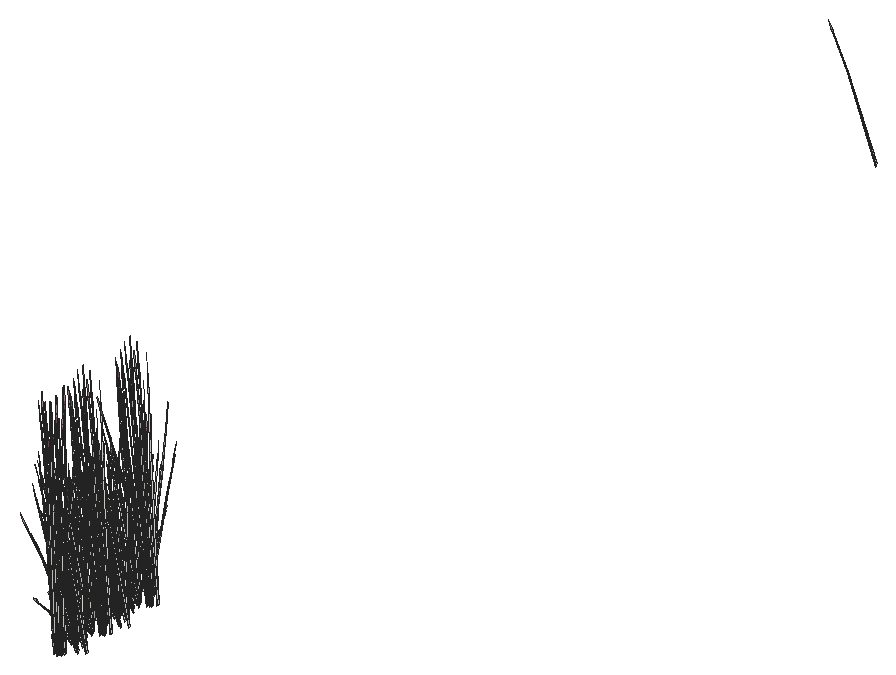
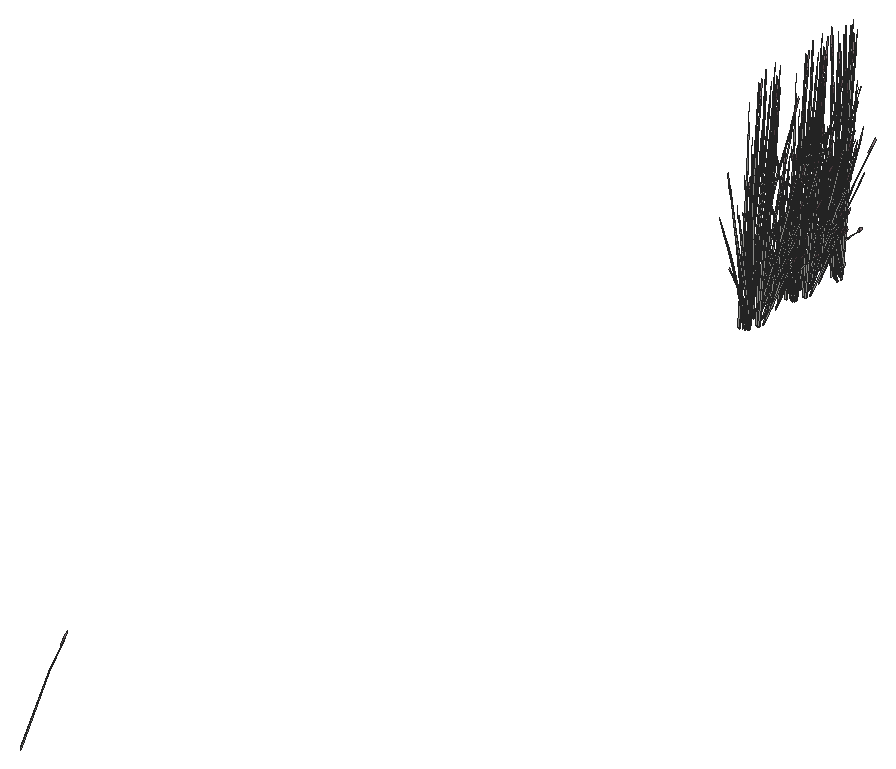
# SketchUp Ruby script. Lengths in inches.
U = 1.inch
M = Sketchup.active_model
def pt(a) = Geom::Point3d.new(a.map { |v| v * U })
def face(e, loops, mat)
  f = e.add_face(loops[0].map { |a| pt(a) })
  loops[1..].each { |l| e.add_face(l.map { |a| pt(a) }).erase! }
  f.material = f.back_material = mat if mat
  f
end
# faces: each face lists its corners as indices into pts; further lists are holes
def faces(e, pts, list, mat = nil) = list.each { |f| face(e, (f[0].is_a?(Array) ? f : [f]).map { |l| l.map { |i| pts[i] } }, mat) }
# xy, xz, yz: faces in a plane at the given z, y or x. An outline is a flat list of corners, or four numbers for a rectangle; further outlines are holes
def ring(l) = l.size == 4 ? [[l[0], l[1]], [l[2], l[1]], [l[2], l[3]], [l[0], l[3]]] : l.each_slice(2).to_a
def flat(e, list, mat, &to3) = list.each { |f| face(e, (f[0].is_a?(Array) ? f : [f]).map { |l| ring(l).map { |u, v| to3.(u, v) } }, mat) }
def xy(e, z, list, mat = nil) = flat(e, list, mat) { |x, y| [x, y, z] }
def xz(e, y, list, mat = nil) = flat(e, list, mat) { |x, z| [x, y, z] }
def yz(e, x, list, mat = nil) = flat(e, list, mat) { |y, z| [x, y, z] }
def lines(e, pts, list) = list.each { |a, b| e.add_line(pt(pts[a]), pt(pts[b])) }
# prism: a flat outline (further loops are holes) pulled along v
def prism(e, loops, v, mat = nil)
  f = face(e, loops, mat); d = Geom::Vector3d.new(v.map { |x| x * U })
  f.pushpull(f.normal.samedirection?(d) ? d.length : -d.length)
end
def box(e, o, s, mat = nil) = prism(e, [[o, [o[0] + s[0], o[1], o[2]], [o[0] + s[0], o[1] + s[1], o[2]], [o[0], o[1] + s[1], o[2]]]], [0, 0, s[2]], mat)
def at(x, y, z, deg = 0) = Geom::Transformation.translation(pt([x, y, z])) * Geom::Transformation.rotation(ORIGIN, Z_AXIS, deg.degrees)
def axes(o, x, y, z) = Geom::Transformation.new([*x, 0, *y, 0, *z, 0, *pt(o).to_a, 1])
def part(name) = M.definitions.add(name)
# library, detail: a bought-in or finely detailed component or shape, given as its bounding box
def library(name, o, s) = part(name).tap { |d| box(d.entities, o, s) }
def detail(e, o, s) = box(e.add_group.entities, o, s)
def put(e, d, t, mat = nil) = e.add_instance(d, t).tap { |i| i.material = mat if mat }
def group(e, t, mat = nil) = e.add_group.tap { |g| g.transformation = t; g.material = mat if mat }.entities
root = M.entities
M.materials.add("LightPink_Translucent").color = [144, 107, 117]
M.materials["LightPink_Translucent"].alpha = 0.75
c1 = part("blade")
p = [[2.15,0.21,22],[0,0.17,0],[0.09,0.45,0],[2.18,0.31,22],[2.29,0.31,22],[0.38,0.45,0],
  [2.48,0.24,33],[2.49,0.24,33],[2.48,0.22,33]]
faces(c1.entities,p,[[0,1,2,3],[4,5,2,3],[6,3,4,7],[8,0,3,6]])
c2 = part("seeds")
p = [[0.3,-0.1,1.38],[-0.01,-0.03,1.59],[-0.01,-0.03,0.03],[0.14,-0.07,-0.07],[0.29,-0.03,3],[0.15,0.01,3.11]]
faces(c2.entities,p,[[0,1,2,3],[1,0,4,5]],"LightPink_Translucent")
c3 = part("blade with seeds")
put(c3.entities,c1,at(0,0,0))
put(c3.entities,c2,axes([2.4,0.25,30.99],[1.5799,-0.05474,1.17369],[-0.12525,1.92788,0.29478],[-0.07173,-0.02425,1.56792]))
put(root,c3,axes([402.9,48.01,-9.7],[0.54955,-0.14427,0.16428],[0.1357,0.53689,0.32672],[-0.04901,-0.07823,1.49371]))
put(root,c3,axes([406.17,50.12,-8.39],[0.18996,0.09365,1.59586],[-0.39312,0.39287,0.12904],[-0.24502,-0.17723,0.68222]))
put(root,c3,axes([403.73,47.88,-9.95],[-0.16686,-0.46861,0],[0.47648,-0.16411,0],[0,0,1.4375]))
put(root,c3,axes([403.41,47.44,-9.5625],[-0.09866,0.48509,0.13483],[-0.48202,-0.0842,-0.38503],[-0.08772,-0.04981,1.18024]))
put(root,c3,axes([404.54,48.04,-9.7],[0.14774,-0.54019,0.16428],[0.54062,0.15287,0.32672],[-0.09339,0.00263,1.49371]))
put(root,c3,axes([407.4375,49.41,-6.94],[-0.34131,0.52108,-0.12682],[-0.49429,-0.3002,-0.70393],[-0.17182,-0.14722,1.06961]))
put(root,c3,axes([403.61,48.1,-9.95],[-0.51557,-0.24403,0],[0.24813,-0.50705,0],[0,0,1.51513]))
put(root,c3,axes([402.72,48.29,-9.69],[0.47863,0.27177,0.46235],[-0.28609,0.48733,0],[-0.10901,-0.0619,1.46668]))
put(root,c3,axes([406.13,49.26,-7.61],[-0.11004,-0.00384,1.62908],[-0.35032,0.38367,-0.25764],[-0.18692,-0.07839,0.13065]))
put(root,c3,axes([404.28,47.08,-9.47],[0.55535,-0.03355,0.41661],[0.05022,0.55698,-0.2005],[-0.09942,0.05645,1.33761]))
put(root,c3,axes([406.05,50.125,-7.26],[0.42234,-0.40113,0.50064],[0.36424,0.42599,0.4128],[-0.19815,-0.07399,1.03595]))
put(root,c3,axes([404.4,48.65,-9.96],[-0.31576,-0.54657,-0.04789],[0.53494,-0.30375,0.48057],[-0.13182,0.05204,1.52373]))
put(root,c3,axes([406.24,50.12,-7.6],[0.02575,-0.41332,0.05988],[0.38885,0.01133,0.47138],[-0.14895,-0.04325,0.71878]))
put(root,c3,axes([404.29,47.32,-9.5625],[0.37783,0.32657,0.13483],[-0.31516,0.36844,-0.38503],[-0.08772,0.04981,1.18024]))
put(root,c3,axes([406.09,50.25,-7.78],[-0.29098,-0.34031,-0.32977],[0.33226,-0.32215,0.42575],[-0.16881,-0.04902,0.81462]))
put(root,c3,axes([405.99,50.61,-9.59],[0.09985,0.15133,1.33163],[-0.23008,0.41134,-0.28638],[-0.23625,-0.09832,0.56934]))
put(root,c3,axes([404.6875,48.33,-9.69],[0.47863,-0.27177,0.46235],[0.28609,0.48733,0],[-0.10901,0.0619,1.46668]))
put(root,c3,axes([404.25,48.58,-10.11],[-0.47712,-0.13449,-0.28847],[0.12013,-0.47362,0.28847],[-0.09619,0.05462,1.29413]))
put(root,c3,axes([406.4,50.48,-7.36],[-0.51122,-0.01309,-0.66157],[0.03434,-0.5511,0.07984],[-0.21658,-0.05816,0.93586]))
put(root,c3,axes([404.17,47.2,-9.52],[0.05959,0.62022,-0.27094],[-0.62068,0.0375,-0.46562],[-0.1093,0.08261,1.4872]))
put(root,c3,axes([405.7,49.58,-7.62],[0.03791,0.05424,1.65179],[-0.18278,0.48761,-0.15608],[-0.18511,0.00353,0.29231]))
put(root,c3,axes([406.23,50.59,-7.64],[-0.37135,0.36005,-0.47583],[-0.32522,-0.38035,-0.36857],[-0.18868,-0.05478,0.91046]))
put(root,c3,axes([406.5,50.43,-7.3],[0.29098,0.34031,0.32977],[-0.33226,0.32215,-0.42575],[-0.16881,-0.04902,0.81462]))
put(root,c3,axes([405.39,51.07,-9.42],[0.3265,-0.03889,1.06958],[-0.20711,0.3427,0.78586],[-0.16135,-0.05141,0.23558]))
put(root,c3,axes([404.41,48.36,-9.83],[0.64025,0.17667,0.2864],[-0.16018,0.63149,-0.33981],[-0.10597,0.07904,1.53541]))
put(root,c3,axes([404.37,48.79,-10.12],[-0.47863,0.27177,-0.46235],[-0.28609,-0.48733,0],[-0.10901,0.0619,1.46668]))
put(root,c3,axes([406.42,50.21,-7.3125],[-0.02738,0.55277,-0.11324],[-0.51847,-0.01511,-0.62851],[-0.19968,-0.0384,0.95501]))
put(root,c3,axes([402.21,48.13,-7.3],[0.34603,-0.28618,0.32977],[0.32756,0.32677,-0.42575],[-0.04984,0.16603,0.81462]))
put(root,c3,axes([404.8,48.71,-9.79],[0.31974,0.54466,0],[-0.53494,0.30375,-0.48057],[-0.12184,0.06918,1.52448]))
put(root,c3,axes([404.53,46.55,-9.35],[-0.01397,-0.51177,1.31553],[0.63227,0.13266,0.557],[-0.14954,0.28003,1.24175]))
put(root,c3,axes([407.34,52.41,-10.08],[-0.53199,-0.08911,-0.58063],[0.11226,-0.54969,-0.15239],[-0.15876,-0.06661,1.28164]))
put(root,c3,axes([405.68,51.38,-7.59],[0.14449,-0.4956,0.447],[0.47502,0.16947,0.36857],[-0.1868,0.02978,0.92496]))
put(root,c3,axes([405.64,51.25,-7.6],[-0.18783,-0.37061,0.05988],[0.34252,-0.1814,0.47138],[-0.15099,0.03579,0.71878]))
put(root,c3,axes([405.63,51.63,-10.61],[0.01297,0.08566,1.6421],[-0.26146,0.44735,-0.25086],[-0.18572,-0.02255,0.2797]))
put(root,c3,axes([404.52,56.44,-8.39],[0.1169,0.17452,1.59586],[-0.54019,0.14692,0.12904],[-0.12209,-0.27397,0.68222]))
put(root,c3,axes([405.58,51.43,-7.78],[-0.42502,-0.15163,-0.32977],[0.12396,-0.44238,0.42575],[-0.17112,0.04056,0.81462]))
put(root,c3,axes([403.04,48.98,-7.6],[-0.37684,0.18473,0.05988],[-0.18445,-0.33686,0.47138],[0.03639,0.14849,0.71878]))
put(root,c3,axes([405.42,55.28,-7.61],[-0.07822,-0.07621,1.62908],[-0.52201,0.04832,-0.25764],[-0.08331,-0.18228,0.13065]))
put(root,c3,axes([401.99,48.21,-6.97],[0.56206,0.02693,-0.12569],[-0.01536,0.50991,-0.69765],[-0.03904,0.19638,1.06006]))
put(root,c3,axes([403.17,48.94,-7.28],[-0.50393,-0.1421,0.49617],[0.17232,-0.46717,0.40911],[0.03028,0.18372,1.0267]))
put(root,c3,axes([404.375,55.98,-9.59],[-0.03097,0.17781,1.33163],[-0.45273,0.14885,-0.28638],[-0.10583,-0.22982,0.56934]))
put(root,c3,axes([403.12,48.87,-10.61],[0.08277,-0.02958,1.6421],[0.49786,0.16279,-0.25086],[0.01456,0.18348,0.2797]))
put(root,c3,axes([402.37,48.4,-7.34],[0.3661,0.36521,-0.52818],[-0.38674,0.31985,-0.40911],[-0.0557,0.18556,1.01061]))
put(root,c3,axes([406.03,51.39,-7.3],[0.42502,0.15163,0.32977],[-0.12396,0.44238,-0.42575],[-0.17112,0.04056,0.81462]))
put(root,c3,axes([401.98,48.95,-9.37],[0.46459,-0.09625,0.0606],[0.10681,0.38778,-0.80367],[-0.02945,0.1963,0.72038]))
put(root,c3,axes([403.23,49.04,-7.78],[-0.15418,0.41799,-0.32977],[-0.44981,-0.12192,0.42575],[0.04124,0.16829,0.81462]))
put(root,c3,axes([406.87,51.36,-8.89],[0.14537,-0.07863,1.64882],[0.05013,0.549,0.12904],[-0.31487,0.07285,0.5893]))
put(root,c3,axes([402.79,47.875,-8.39],[-0.01252,-0.20862,1.59586],[0.54251,0.1384,0.12904],[-0.03356,0.2973,0.68222]))
put(root,c3,axes([404.88,55.03,-7.62],[-0.00954,0.06515,1.65179],[-0.47055,0.23645,-0.15608],[-0.13847,-0.12087,0.29231]))
put(root,c3,axes([405.31,51.73,-7.61],[-0.08351,0.07057,1.62908],[0.0071,0.51561,-0.25764],[-0.19143,0.06705,0.13065]))
put(root,c3,axes([405.87,51.66,-7.64],[-0.13855,0.49442,-0.47583],[-0.47502,-0.16947,-0.36857],[-0.19125,0.04534,0.91046]))
put(root,c3,axes([405.85,51.24,-7.3125],[0.25732,0.49218,-0.11324],[-0.45669,0.24187,-0.62851],[-0.19245,0.06494,0.95501]))
put(root,c3,axes([404.78,56.19,-7.26],[0.56969,-0.13971,0.50064],[0.09887,0.54803,0.4128],[-0.13398,-0.16152,1.03595]))
put(root,c3,axes([404.22,55.69,-9.42],[0.26677,0.18918,1.06958],[-0.38851,0.11372,0.78586],[-0.08313,-0.14539,0.23558]))
put(root,c3,axes([404.86,56.7,-7.36],[-0.43608,-0.26272,-0.66157],[0.30991,-0.46038,0.07984],[-0.158,-0.15687,0.93586]))
put(root,c3,axes([404.71,56.35,-7.78],[-0.07899,-0.43781,-0.32977],[0.45153,-0.11561,0.42575],[-0.12128,-0.12546,0.81462]))
put(root,c3,axes([404.91,56.31,-7.6],[0.23243,-0.34529,0.05988],[0.331,0.20103,0.47138],[-0.10701,-0.1107,0.71878]))
put(root,c3,axes([404.01,56.26,-10.61],[-0.04954,0.0716,1.6421],[-0.50062,0.15438,-0.25086],[-0.12094,-0.14044,0.2797]))
put(root,c3,axes([402.07,48.9375,-8.87],[0.01124,-0.2806,1.43727],[0.50537,0.14821,0.19862],[-0.04379,0.29905,0.67868]))
put(root,c3,axes([405.79,52.61,-7.59],[-0.12683,-0.50025,0.447],[0.49754,-0.08682,0.36857],[-0.14663,0.11765,0.92496]))
put(root,c3,axes([405.69,52.52,-7.6],[-0.35109,-0.22859,0.05988],[0.2044,-0.32553,0.47138],[-0.11256,0.10524,0.71878]))
put(root,c3,axes([404.66,56.71,-7.64],[-0.50465,0.12921,-0.47583],[-0.08828,-0.48932,-0.36857],[-0.13555,-0.14022,0.91046]))
put(root,c3,axes([404.38,52.25,-7.62],[0.06527,0.01458,1.65179],[0.20191,0.48025,-0.15608],[-0.1336,0.12605,0.29231]))
put(root,c3,axes([404.93,53.77,-9.42],[0.21313,-0.24635,1.06958],[0.0841,0.38999,0.78586],[-0.15402,0.06983,0.23558]))
put(root,c3,axes([405.73,52.71,-7.78],[-0.44516,0.07768,-0.32977],[-0.11755,-0.44407,0.42575],[-0.12757,0.11927,0.81462]))
put(root,c3,axes([405.91,59.67,-8.9],[0.44194,0.21918,1.40854],[-0.43295,0.47219,0.557],[-0.19393,-0.27986,1.18082]))
put(root,c3,axes([404.98,56.7,-7.3],[0.07899,0.43781,0.32977],[-0.45153,0.11561,-0.42575],[-0.12128,-0.12546,0.81462]))
put(root,c3,axes([403.6,58.15,-10.12],[0,-0.54355,-0.46235],[0.57217,0,0],[0,-0.1238,1.46668]))
put(root,c3,axes([403.7,56.54,-10.02],[-0.14753,0.44383,-0.03625],[-0.45406,-0.13653,-0.16435],[-0.06894,-0.07259,0.54209]))
put(root,c3,axes([406.5,52.27,-8.39],[0.12773,-0.16701,1.59586],[0.32252,0.4508,0.12904],[-0.22121,0.20529,0.68222]))
put(root,c3,axes([406.1,52.76,-7.64],[0.13138,0.49631,-0.47583],[-0.49754,0.08682,-0.36857],[-0.14258,0.13331,0.91046]))
put(root,c3,axes([403.45,58.56,-9.79],[-0.63949,0,0],[0,-0.60749,-0.48057],[0,-0.13836,1.52448]))
put(root,c3,axes([405.49,54.03,-10.61],[0.0686,0.0543,1.6421],[0.11632,0.50315,-0.25086],[-0.15204,0.10729,0.2797]))
put(root,c3,axes([403.95,58.4,-9.83],[-0.47569,0.45698,0.2864],[-0.47598,-0.45217,-0.33981],[-0.01661,-0.12977,1.53541]))
put(root,c3,axes([405.24,59.36,-9.73],[0.13555,-0.64407,-0.21817],[0.64269,0.11227,0.47743],[-0.1123,-0.08895,1.45677]))
put(root,c3,axes([406.41,52.68,-8.39],[0.09522,-0.18683,1.59586],[0.39947,0.38663,0.12904],[-0.18021,0.24097,0.68222]))
put(root,c3,axes([404.08,57.3,-7.3],[0.29098,0.34031,0.32977],[-0.33226,0.32215,-0.42575],[-0.16881,-0.04902,0.81462]))
put(root,c3,axes([405.32,53.65,-7.61],[-0.01271,0.10756,1.62908],[0.36076,0.37419,-0.25764],[-0.09444,0.17695,0.13065]))
put(root,c3,axes([403.84,58.66,-9.69],[0,0.54355,0.46235],[-0.57217,0,0],[0,-0.1238,1.46668]))
put(root,c3,axes([405.19,59.1,-9.94],[-0.30722,-0.45622,-0.41661],[0.46535,-0.32126,0.2005],[-0.09942,-0.05645,1.33761]))
put(root,c3,axes([404.35,60.11,-10.11],[-0.12013,-0.47362,-0.28847],[0.47712,-0.13449,0.28847],[-0.09619,-0.05462,1.29413]))
put(root,c3,axes([404.22,60.3125,-10.12],[-0.47863,-0.27177,-0.46235],[0.28609,-0.48733,0],[-0.10901,-0.0619,1.46668]))
put(root,c3,axes([405.52,59.35,-9.52],[-0.51635,0.36087,-0.27094],[-0.34336,-0.5099,-0.46562],[-0.1274,-0.05178,1.4872]))
put(root,c3,axes([405.47,59.51,-9.5625],[-0.09866,0.48509,0.13483],[-0.48202,-0.0842,-0.38503],[-0.08772,-0.04981,1.18024]))
put(root,c3,axes([406.1,59.52,-9.7],[-0.49938,-0.43748,-0.23459],[0.42021,-0.49126,0.51337],[-0.13447,0.05118,1.56642]))
put(root,c3,axes([404.79,60.35,-9.69],[0.47863,0.27177,0.46235],[-0.28609,0.48733,0],[-0.10901,-0.0619,1.46668]))
put(root,c3,axes([406.18,62.96,-8.39],[0.18996,0.09365,1.59586],[-0.39312,0.39287,0.12904],[-0.24502,-0.17723,0.68222]))
put(root,c3,axes([404.51,60.64,-9.79],[-0.31974,0.54466,0],[-0.53494,-0.30375,-0.48057],[-0.12184,-0.06918,1.52448]))
put(root,c3,axes([407.45,62.25,-6.94],[-0.34131,0.52108,-0.12682],[-0.49429,-0.3002,-0.70393],[-0.17182,-0.14722,1.06961]))
put(root,c3,axes([405.85,59.42,-9.94],[-0.55535,0.03355,-0.41661],[-0.05022,-0.55698,0.2005],[-0.09942,0.05645,1.33761]))
put(root,c3,axes([406.14,62.1,-7.61],[-0.11004,-0.00384,1.62908],[-0.35032,0.38367,-0.25764],[-0.18692,-0.07839,0.13065]))
put(root,c3,axes([406.46,60.71,-9.96],[-0.31576,-0.54657,-0.04789],[0.53494,-0.30375,0.48057],[-0.13182,0.05204,1.52373]))
put(root,c3,axes([406.06,62.97,-7.26],[0.42234,-0.40113,0.50064],[0.36424,0.42599,0.4128],[-0.19815,-0.07399,1.03595]))
put(root,c3,axes([403.67,59.3125,-7.3],[0.44516,-0.07768,0.32977],[0.11755,0.44407,-0.42575],[-0.12757,0.11927,0.81462]))
put(root,c3,axes([406.25,62.96,-7.6],[0.02575,-0.41332,0.05988],[0.38885,0.01133,0.47138],[-0.14895,-0.04325,0.71878]))
put(root,c3,axes([406.1,63.09,-7.78],[-0.29098,-0.34031,-0.32977],[0.33226,-0.32215,0.42575],[-0.16881,-0.04902,0.81462]))
put(root,c3,axes([406,63.46,-9.59],[0.09985,0.15133,1.33163],[-0.23008,0.41134,-0.28638],[-0.23625,-0.09832,0.56934]))
put(root,c3,axes([402.66,60.57,-6.74],[0.45129,0.14509,-0.06041],[-0.13882,0.44656,-0.27392],[-0.07381,0.0678,0.90349]))
put(root,c3,axes([405.86,59.75,-10.08],[-0.34446,0.40855,-0.58063],[-0.42791,-0.37046,-0.15239],[-0.13803,0.10191,1.28164]))
put(root,c3,axes([406.41,63.32,-7.36],[-0.51122,-0.01309,-0.66157],[0.03434,-0.5511,0.07984],[-0.21658,-0.05816,0.93586]))
put(root,c3,axes([406.43,60.86,-10.12],[-0.47863,0.27177,-0.46235],[-0.28609,-0.48733,0],[-0.10901,0.0619,1.46668]))
put(root,c3,axes([403.44,59.27,-7.3125],[0.47307,0.29971,-0.11324],[-0.27254,0.43404,-0.62851],[-0.13365,0.15087,0.95501]))
put(root,c3,axes([405.72,62.42,-7.62],[0.03791,0.05424,1.65179],[-0.18278,0.48761,-0.15608],[-0.18511,0.00353,0.29231]))
put(root,c3,axes([406.24,63.43,-7.64],[-0.37135,0.36005,-0.47583],[-0.32522,-0.38035,-0.36857],[-0.18868,-0.05478,0.91046]))
put(root,c3,axes([406.51,63.27,-7.3],[0.29098,0.34031,0.32977],[-0.33226,0.32215,-0.42575],[-0.16881,-0.04902,0.81462]))
put(root,c3,axes([405.4,63.91,-9.42],[0.3265,-0.03889,1.06958],[-0.20711,0.3427,0.78586],[-0.16135,-0.05141,0.23558]))
put(root,c3,axes([403.96,60.46,-7.6],[-0.42027,-0.02533,0.05988],[0.01152,-0.38243,0.47138],[-0.04398,0.14649,0.71878]))
put(root,c3,axes([404.09,60.49,-7.59],[-0.36417,-0.37086,0.447],[0.38674,-0.31985,0.36857],[-0.06718,0.174,0.92496]))
put(root,c3,axes([406.43,63.06,-7.3125],[-0.02738,0.55277,-0.11324],[-0.51847,-0.01511,-0.62851],[-0.19968,-0.0384,0.95501]))
put(root,c3,axes([407.35,65.25,-10.08],[-0.53199,-0.08911,-0.58063],[0.11226,-0.54969,-0.15239],[-0.15876,-0.06661,1.28164]))
put(root,c3,axes([404.09,60.6,-7.78],[-0.34603,0.28618,-0.32977],[-0.32756,-0.32677,0.42575],[-0.04984,0.16603,0.81462]))
put(root,c3,axes([405.6875,64.22,-7.59],[0.14449,-0.4956,0.447],[0.47502,0.16947,0.36857],[-0.1868,0.02978,0.92496]))
put(root,c3,axes([404.3125,61.71,-9.42],[-0.01324,-0.32319,1.06958],[0.33072,0.23052,0.78586],[-0.06504,0.15405,0.23558]))
put(root,c3,axes([405.65,64.09,-7.6],[-0.18783,-0.37061,0.05988],[0.34252,-0.1814,0.47138],[-0.15099,0.03579,0.71878]))
put(root,c3,axes([405.64,64.47,-10.61],[0.01297,0.08566,1.6421],[-0.26146,0.44735,-0.25086],[-0.18572,-0.02255,0.2797]))
put(root,c3,axes([405.59,64.27,-7.78],[-0.42502,-0.15163,-0.32977],[0.12396,-0.44238,0.42575],[-0.17112,0.04056,0.81462]))
put(root,c3,axes([404.32,60.3,-7.03],[-0.01331,0.50278,-0.73435],[-0.56035,-0.03377,0.08862],[-0.05914,0.213,1.03881]))
put(root,c3,axes([402.86,61.62,-7.62],[0.05802,-0.03282,1.65179],[0.47954,0.21828,-0.15608],[-0.01127,0.18175,0.29231]))
put(root,c3,axes([406.04,64.23,-7.3],[0.42502,0.15163,0.32977],[-0.12396,0.44238,-0.42575],[-0.17112,0.04056,0.81462]))
put(root,c3,axes([403.93,61.43,-9.59],[0.16138,-0.08575,1.33163],[0.39845,0.25854,-0.28638],[-0.1186,0.22371,0.56934]))
put(root,c3,axes([406.88,64.2,-8.89],[0.14537,-0.07863,1.64882],[0.05013,0.549,0.12904],[-0.31487,0.07285,0.5893]))
put(root,c3,axes([405.32,64.57,-7.61],[-0.08351,0.07057,1.62908],[0.0071,0.51561,-0.25764],[-0.19143,0.06705,0.13065]))
put(root,c3,axes([405.88,64.5,-7.64],[-0.13855,0.49442,-0.47583],[-0.47502,-0.16947,-0.36857],[-0.19125,0.04534,0.91046]))
put(root,c3,axes([404.52,70.68,-8.39],[0.1169,0.17452,1.59586],[-0.54019,0.14692,0.12904],[-0.12209,-0.27397,0.68222]))
put(root,c3,axes([405.86,64.08,-7.3125],[0.25732,0.49218,-0.11324],[-0.45669,0.24187,-0.62851],[-0.19245,0.06494,0.95501]))
put(root,c3,axes([404.14,61.01,-8.87],[0.01124,-0.2806,1.43727],[0.50537,0.14821,0.19862],[-0.04379,0.29905,0.67868]))
put(root,c3,axes([405.41,69.53,-7.61],[-0.07822,-0.07621,1.62908],[-0.52201,0.04832,-0.25764],[-0.08331,-0.18228,0.13065]))
put(root,c3,axes([404.37,70.22,-9.59],[-0.03097,0.17781,1.33163],[-0.45273,0.14885,-0.28638],[-0.10583,-0.22982,0.56934]))
put(root,c3,axes([405.8,65.45,-7.59],[-0.12683,-0.50025,0.447],[0.49754,-0.08682,0.36857],[-0.14663,0.11765,0.92496]))
put(root,c3,axes([405.7,65.36,-7.6],[-0.35109,-0.22859,0.05988],[0.2044,-0.32553,0.47138],[-0.11256,0.10524,0.71878]))
put(root,c3,axes([404.875,69.28,-7.62],[-0.00954,0.06515,1.65179],[-0.47055,0.23645,-0.15608],[-0.13847,-0.12087,0.29231]))
put(root,c3,axes([404.77,70.43,-7.26],[0.56969,-0.13971,0.50064],[0.09887,0.54803,0.4128],[-0.13398,-0.16152,1.03595]))
put(root,c3,axes([404.39,65.09,-7.62],[0.06527,0.01458,1.65179],[0.20191,0.48025,-0.15608],[-0.1336,0.12605,0.29231]))
put(root,c3,axes([404.21,69.9375,-9.42],[0.26677,0.18918,1.06958],[-0.38851,0.11372,0.78586],[-0.08313,-0.14539,0.23558]))
put(root,c3,axes([404.94,66.62,-9.42],[0.21313,-0.24635,1.06958],[0.0841,0.38999,0.78586],[-0.15402,0.06983,0.23558]))
put(root,c3,axes([404.86,70.9375,-7.36],[-0.43608,-0.26272,-0.66157],[0.30991,-0.46038,0.07984],[-0.158,-0.15687,0.93586]))
put(root,c3,axes([404.71,70.59,-7.78],[-0.07899,-0.43781,-0.32977],[0.45153,-0.11561,0.42575],[-0.12128,-0.12546,0.81462]))
put(root,c3,axes([405.74,65.55,-7.78],[-0.44516,0.07768,-0.32977],[-0.11755,-0.44407,0.42575],[-0.12757,0.11927,0.81462]))
put(root,c3,axes([404.9,70.55,-7.6],[0.23243,-0.34529,0.05988],[0.331,0.20103,0.47138],[-0.10701,-0.1107,0.71878]))
put(root,c3,axes([404,70.51,-10.61],[-0.04954,0.0716,1.6421],[-0.50062,0.15438,-0.25086],[-0.12094,-0.14044,0.2797]))
put(root,c3,axes([404.65,70.95,-7.64],[-0.50465,0.12921,-0.47583],[-0.08828,-0.48932,-0.36857],[-0.13555,-0.14022,0.91046]))
put(root,c3,axes([406.51,65.11,-8.39],[0.12773,-0.16701,1.59586],[0.32252,0.4508,0.12904],[-0.22121,0.20529,0.68222]))
put(root,c3,axes([406.11,65.6,-7.64],[0.13138,0.49631,-0.47583],[-0.49754,0.08682,-0.36857],[-0.14258,0.13331,0.91046]))
put(root,c3,axes([405.5,66.87,-10.61],[0.0686,0.0543,1.6421],[0.11632,0.50315,-0.25086],[-0.15204,0.10729,0.2797]))
put(root,c3,axes([405.9,73.91,-8.9],[0.44194,0.21918,1.40854],[-0.43295,0.47219,0.557],[-0.19393,-0.27986,1.18082]))
put(root,c3,axes([404.97,70.95,-7.3],[0.07899,0.43781,0.32977],[-0.45153,0.11561,-0.42575],[-0.12128,-0.12546,0.81462]))
put(root,c3,axes([403.59,72.4,-10.12],[0,-0.54355,-0.46235],[0.57217,0,0],[0,-0.1238,1.46668]))
put(root,c3,axes([406.42,65.53,-8.39],[0.09522,-0.18683,1.59586],[0.39947,0.38663,0.12904],[-0.18021,0.24097,0.68222]))
put(root,c3,axes([405.33,66.49,-7.61],[-0.01271,0.10756,1.62908],[0.36076,0.37419,-0.25764],[-0.09444,0.17695,0.13065]))
put(root,c3,axes([403.69,70.78,-10.02],[-0.14753,0.44383,-0.03625],[-0.45406,-0.13653,-0.16435],[-0.06894,-0.07259,0.54209]))
put(root,c3,axes([403.45,72.81,-9.79],[-0.63949,0,0],[0,-0.60749,-0.48057],[0,-0.13836,1.52448]))
put(root,c3,axes([403.94,72.65,-9.83],[-0.47569,0.45698,0.2864],[-0.47598,-0.45217,-0.33981],[-0.01661,-0.12977,1.53541]))
put(root,c3,axes([405.23,73.6,-9.73],[0.13555,-0.64407,-0.21817],[0.64269,0.11227,0.47743],[-0.1123,-0.08895,1.45677]))
put(root,c3,axes([404.07,71.54,-7.3],[0.29098,0.34031,0.32977],[-0.33226,0.32215,-0.42575],[-0.16881,-0.04902,0.81462]))
put(root,c3,axes([403.84,72.9,-9.69],[0,0.54355,0.46235],[-0.57217,0,0],[0,-0.1238,1.46668]))
put(root,c3,axes([405.1875,73.34,-9.94],[-0.30722,-0.45622,-0.41661],[0.46535,-0.32126,0.2005],[-0.09942,-0.05645,1.33761]))
put(root,c3,axes([404.35,74.35,-10.11],[-0.12013,-0.47362,-0.28847],[0.47712,-0.13449,0.28847],[-0.09619,-0.05462,1.29413]))
put(root,c3,axes([404.21,74.55,-10.12],[-0.47863,-0.27177,-0.46235],[0.28609,-0.48733,0],[-0.10901,-0.0619,1.46668]))
put(root,c3,axes([405.51,73.6,-9.52],[-0.51635,0.36087,-0.27094],[-0.34336,-0.5099,-0.46562],[-0.1274,-0.05178,1.4872]))
put(root,c3,axes([405.46,73.75,-9.5625],[-0.09866,0.48509,0.13483],[-0.48202,-0.0842,-0.38503],[-0.08772,-0.04981,1.18024]))
put(root,c3,axes([406.09,73.76,-9.7],[-0.49938,-0.43748,-0.23459],[0.42021,-0.49126,0.51337],[-0.13447,0.05118,1.56642]))
put(root,c3,axes([404.78,74.6,-9.69],[0.47863,0.27177,0.46235],[-0.28609,0.48733,0],[-0.10901,-0.0619,1.46668]))
put(root,c3,axes([404.5,74.88,-9.79],[-0.31974,0.54466,0],[-0.53494,-0.30375,-0.48057],[-0.12184,-0.06918,1.52448]))
put(root,c3,axes([405.84,73.67,-9.94],[-0.55535,0.03355,-0.41661],[-0.05022,-0.55698,0.2005],[-0.09942,0.05645,1.33761]))
put(root,c3,axes([406.46,74.96,-9.96],[-0.31576,-0.54657,-0.04789],[0.53494,-0.30375,0.48057],[-0.13182,0.05204,1.52373]))
put(root,c3,axes([403.67,73.56,-7.3],[0.44516,-0.07768,0.32977],[0.11755,0.44407,-0.42575],[-0.12757,0.11927,0.81462]))
put(root,c3,axes([402.66,74.82,-6.74],[0.45129,0.14509,-0.06041],[-0.13882,0.44656,-0.27392],[-0.07381,0.0678,0.90349]))
put(root,c3,axes([405.86,73.99,-10.08],[-0.34446,0.40855,-0.58063],[-0.42791,-0.37046,-0.15239],[-0.13803,0.10191,1.28164]))
put(root,c3,axes([406.42,75.1,-10.12],[-0.47863,0.27177,-0.46235],[-0.28609,-0.48733,0],[-0.10901,0.0619,1.46668]))
put(root,c3,axes([403.44,73.52,-7.3125],[0.47307,0.29971,-0.11324],[-0.27254,0.43404,-0.62851],[-0.13365,0.15087,0.95501]))
put(root,c3,axes([403.95,74.7,-7.6],[-0.42027,-0.02533,0.05988],[0.01152,-0.38243,0.47138],[-0.04398,0.14649,0.71878]))
put(root,c3,axes([404.09,74.74,-7.59],[-0.36417,-0.37086,0.447],[0.38674,-0.31985,0.36857],[-0.06718,0.174,0.92496]))
put(root,c3,axes([404.09,74.85,-7.78],[-0.34603,0.28618,-0.32977],[-0.32756,-0.32677,0.42575],[-0.04984,0.16603,0.81462]))
put(root,c3,axes([404.31,75.96,-9.42],[-0.01324,-0.32319,1.06958],[0.33072,0.23052,0.78586],[-0.06504,0.15405,0.23558]))
put(root,c3,axes([404.32,74.54,-7.03],[-0.01331,0.50278,-0.73435],[-0.56035,-0.03377,0.08862],[-0.05914,0.213,1.03881]))
put(root,c3,axes([402.85,75.86,-7.62],[0.05802,-0.03282,1.65179],[0.47954,0.21828,-0.15608],[-0.01127,0.18175,0.29231]))
put(root,c3,axes([403.92,75.67,-9.59],[0.16138,-0.08575,1.33163],[0.39845,0.25854,-0.28638],[-0.1186,0.22371,0.56934]))
put(root,c3,axes([404.13,75.25,-8.87],[0.01124,-0.2806,1.43727],[0.50537,0.14821,0.19862],[-0.04379,0.29905,0.67868]))
put(root,c3,axes([408.62,289.34,-8.39],[0.21212,-0.01231,1.59586],[-0.14072,0.53355,0.12904],[-0.3023,-0.033,0.68222]))
